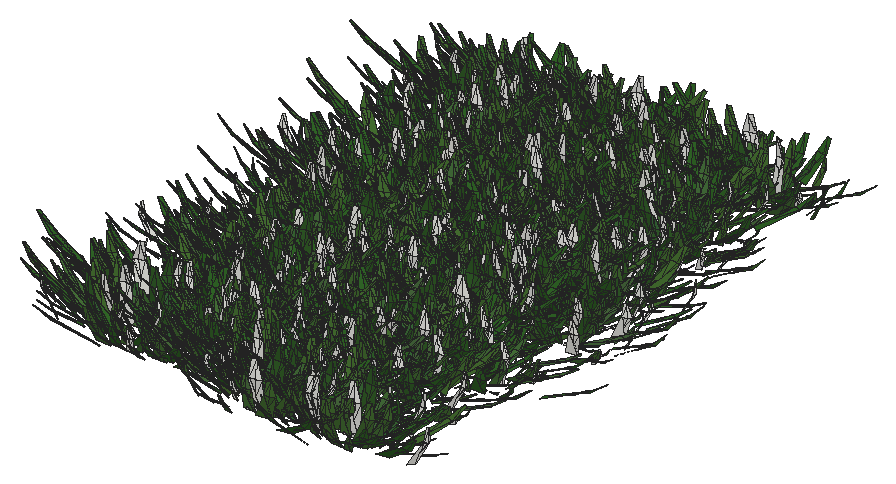
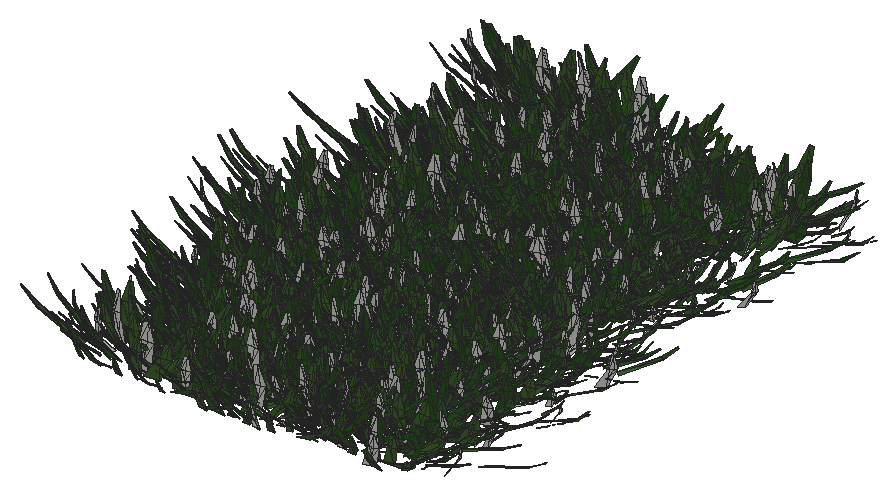
# SketchUp Ruby script. Lengths in inches.
U = 1.inch
M = Sketchup.active_model
def pt(a) = Geom::Point3d.new(a.map { |v| v * U })
def face(e, loops, mat)
  f = e.add_face(loops[0].map { |a| pt(a) })
  loops[1..].each { |l| e.add_face(l.map { |a| pt(a) }).erase! }
  f.material = f.back_material = mat if mat
  f
end
# faces: each face lists its corners as indices into pts; further lists are holes
def faces(e, pts, list, mat = nil) = list.each { |f| face(e, (f[0].is_a?(Array) ? f : [f]).map { |l| l.map { |i| pts[i] } }, mat) }
# xy, xz, yz: faces in a plane at the given z, y or x. An outline is a flat list of corners, or four numbers for a rectangle; further outlines are holes
def ring(l) = l.size == 4 ? [[l[0], l[1]], [l[2], l[1]], [l[2], l[3]], [l[0], l[3]]] : l.each_slice(2).to_a
def flat(e, list, mat, &to3) = list.each { |f| face(e, (f[0].is_a?(Array) ? f : [f]).map { |l| ring(l).map { |u, v| to3.(u, v) } }, mat) }
def xy(e, z, list, mat = nil) = flat(e, list, mat) { |x, y| [x, y, z] }
def xz(e, y, list, mat = nil) = flat(e, list, mat) { |x, z| [x, y, z] }
def yz(e, x, list, mat = nil) = flat(e, list, mat) { |y, z| [x, y, z] }
def lines(e, pts, list) = list.each { |a, b| e.add_line(pt(pts[a]), pt(pts[b])) }
# prism: a flat outline (further loops are holes) pulled along v
def prism(e, loops, v, mat = nil)
  f = face(e, loops, mat); d = Geom::Vector3d.new(v.map { |x| x * U })
  f.pushpull(f.normal.samedirection?(d) ? d.length : -d.length)
end
def box(e, o, s, mat = nil) = prism(e, [[o, [o[0] + s[0], o[1], o[2]], [o[0] + s[0], o[1] + s[1], o[2]], [o[0], o[1] + s[1], o[2]]]], [0, 0, s[2]], mat)
def at(x, y, z, deg = 0) = Geom::Transformation.translation(pt([x, y, z])) * Geom::Transformation.rotation(ORIGIN, Z_AXIS, deg.degrees)
def axes(o, x, y, z) = Geom::Transformation.new([*x, 0, *y, 0, *z, 0, *pt(o).to_a, 1])
def part(name) = M.definitions.add(name)
# library, detail: a bought-in or finely detailed component or shape, given as its bounding box
def library(name, o, s) = part(name).tap { |d| box(d.entities, o, s) }
def detail(e, o, s) = box(e.add_group.entities, o, s)
def put(e, d, t, mat = nil) = e.add_instance(d, t).tap { |i| i.material = mat if mat }
def group(e, t, mat = nil) = e.add_group.tap { |g| g.transformation = t; g.material = mat if mat }.entities
root = M.entities
M.materials.add("Material82").color = [68, 110, 58]
M.materials.add("Material83").color = [48, 90, 38]
M.materials.add("Material84").color = [68, 110, 48]
M.materials.add("Material85").color = [48, 90, 48]
M.materials.add("Material86").color = [58, 110, 58]
M.materials.add("Material87").color = [58, 90, 38]
M.materials.add("Material88").color = [68, 100, 58]
M.materials.add("Material89").color = [48, 100, 38]
c1 = part("grass00")
p = [[-0.6875,0.15,0],[-0.56,0.08,5.52],[-0.04,0.03,2.76],[0.48,-0.02,0],[0.35,-0.02,5.52],[-0.1,-0.14,5.52],
  [-0.12,0.65,8.37],[-0.42,0.65,8.37]]
faces(c1.entities,p,[[0,1,2,3],[3,2,4],[1,5,2],[5,4,2],[1,6,5],[4,5,6],[7,6,1]])
c2 = part("Group16\#1")
put(c2.entities,c1,axes([1.44,-0.61,-0.01],[0.05352,0.12609,0],[-0.10704,0.04543,0.07239],[0.06664,-0.02828,0.11628]),"Material85")
put(c2.entities,c1,axes([0.76,-0.15,-0.01],[0.04676,0.24062,0],[-0.23162,0.04501,0.06642],[0.0652,-0.01267,0.23595]),"Material82")
put(c2.entities,c1,axes([0.79,0.01,-0.01],[-0.00606,0.34651,0],[-0.34381,-0.00602,0.0432],[0.04319,0.00076,0.34386]))
put(c2.entities,c1,axes([1,0.23,-0.01],[-0.07192,0.31144,0],[-0.28722,-0.06632,0.1236],[0.12043,0.02781,0.29478]),"Material84")
put(c2.entities,c1,axes([1.66,0.77,-0.01],[-0.13828,0.29651,0],[-0.21551,-0.1005,0.22471],[0.20365,0.09498,0.23779]),"Material89")
put(c2.entities,c1,axes([0.6875,0.52,-0.01],[-0.18126,0.24051,0],[-0.22746,-0.17142,0.09788],[0.07817,0.05891,0.28481]),"Material84")
put(c2.entities,c1,axes([0.68,0.78,-0.01],[-0.215,0.18688,0],[-0.12385,-0.14248,0.21334],[0.13995,0.16101,0.18878]),"Material82")
put(c2.entities,c1,axes([0.56,1,-0.01],[-0.13756,0.07624,0],[-0.06159,-0.11112,0.0927],[0.04494,0.08108,0.12705]),"Material84")
put(c2.entities,c1,axes([0.2,0.64,-0.01],[-0.23729,0.07254,0],[-0.05711,-0.18681,0.153],[0.04473,0.14632,0.19535]),"Material89")
put(c2.entities,c1,axes([0.0625,0.72,-0.01],[-0.28874,0.02525,0],[-0.02179,-0.24916,0.14647],[0.01276,0.14591,0.25012]),"Material82")
put(c2.entities,c1,axes([-0.08,0.62,-0.01],[-0.34089,-0.04187,0],[0.03255,-0.26504,0.216],[-0.02633,0.21439,0.26703]),"Material89")
put(c2.entities,c1,axes([-0.34,0.98,-0.01],[-0.14314,-0.0493,0],[0.04397,-0.12769,0.06843],[-0.02228,0.0647,0.13505]),"Material89")
put(c2.entities,c1,axes([-0.87,1.45,-0.01],[-0.23488,-0.14114,0],[0.13761,-0.22901,0.06087],[-0.03135,0.05217,0.26717]))
put(c2.entities,c1,axes([-0.72,0.77,-0.01],[-0.14208,-0.13251,0],[0.07209,-0.0773,0.16301],[-0.11118,0.11922,0.1057]),"Material89")
put(c2.entities,c1,axes([-0.62,0.43,-0.01],[-0.14845,-0.21203,0],[0.18654,-0.13061,0.12304],[-0.10079,0.07057,0.22772]),"Material82")
put(c2.entities,c1,axes([-0.68,0.29,-0.01],[-0.13639,-0.32136,0],[0.31723,-0.13464,0.05579],[-0.05136,0.0218,0.34462]),"Material83")
put(c2.entities,c1,axes([-0.64,0.125,-0.01],[-0.0458,-0.23569,0],[0.22124,-0.043,0.08276],[-0.08124,0.01579,0.22538]),"Material86")
put(c2.entities,c1,axes([-1.6,-0.03,-0.01],[0.00576,-0.32897,0],[0.27526,0.00482,0.18018],[-0.18015,-0.00315,0.2753]),"Material84")
put(c2.entities,c1,axes([-1.36,-0.31,-0.01],[0.05718,-0.24765,0],[0.18172,0.04196,0.17267],[-0.16825,-0.03885,0.1865]),"Material89")
put(c2.entities,c1,axes([-1.54,-0.72,-0.01],[0.06537,-0.14017,0],[0.13555,0.06321,0.03939],[-0.0357,-0.01665,0.14956]))
put(c2.entities,c1,axes([-1.19,-0.9,-0.01],[0.09597,-0.12735,0],[0.11214,0.08451,0.07557],[-0.06035,-0.04548,0.14042]),"Material88")
put(c2.entities,c1,axes([-0.47,-0.54,-0.01],[0.11588,-0.10072,0],[0.0618,0.0711,0.12124],[-0.07953,-0.0915,0.0942]))
put(c2.entities,c1,axes([-0.47,-0.84,-0.01],[0.11927,-0.0661,0],[0.06603,0.11913,0.00646],[-0.00313,-0.00565,0.13621]),"Material84")
put(c2.entities,c1,axes([-0.38,-1.24,-0.01],[0.28037,-0.08571,0],[0.0618,0.20215,0.20315],[-0.05939,-0.19428,0.21139]),"Material88")
put(c2.entities,c1,axes([-0.06,-0.66,-0.01],[0.22719,-0.01987,0],[0.01247,0.14255,0.17758],[-0.01547,-0.17691,0.1431]),"Material87")
put(c2.entities,c1,axes([0.11,-0.89,-0.01],[0.14882,0.01828,0],[-0.01058,0.08611,0.12229],[0.01491,-0.12138,0.08676]),"Material85")
put(c2.entities,c1,axes([0.25,-0.72,-0.01],[0.20481,0.07053,0],[-0.06206,0.18022,0.10291],[0.03351,-0.0973,0.1906]),"Material85")
put(c2.entities,c1,axes([0.85,-1.42,-0.01],[0.16481,0.09904,0],[-0.09472,0.15762,0.05616],[0.02893,-0.04814,0.18389]),"Material84")
put(c2.entities,c1,axes([1.01,-1.09,-0.01],[0.21858,0.20385,0],[-0.17495,0.1876,0.15339],[0.10462,-0.11218,0.25652]),"Material89")
put(c2.entities,c1,axes([1.01,-0.71,-0.01],[0.08733,0.12473,0],[-0.06445,0.04512,0.13037],[0.1068,-0.07477,0.07867]),"Material85")
c3 = part("Group15\#1")
put(c3.entities,c2,at(0,0,0))
c4 = part("3darcstudiotree_grass00\#1")
put(c4.entities,c3,at(0,0,0))
put(root,c4,axes([1704.59,960.15,-29.74],[-3.29694,-0.59268,0],[1.38855,-1.20133,-0.0331],[0.08455,-0.07315,1.54531]))
put(root,c4,axes([1703.45,956.93,-29.74],[2.67683,1.25305,0],[-2.64635,0.87925,-0.04423],[-0.18001,0.05981,1.38013]))
put(root,c4,axes([1704.59,979.83,-29.74],[1.85229,-1.14191,0],[3.43107,0.86561,-0.02581],[0.11483,0.02897,1.61243]))
put(root,c4,axes([1705.09,970.66,-29.74],[-0.72323,-1.62263,0],[3.80365,-0.26368,-0.04893],[0.28769,-0.01994,1.72817]))
put(root,c4,axes([1704.83,992.4,-29.74],[-3.72731,0.81099,0],[-1.84954,-1.32207,-0.01481],[-0.0358,-0.02559,1.43556]))
put(root,c4,axes([1704.18,984.05,-29.74],[4.17155,-0.17702,0],[0.50263,1.84221,-0.03237],[0.01504,0.05512,1.52951]))
put(root,c4,axes([1705.72,951.16,-29.74],[-4.25916,-0.67423,0],[1.26133,-1.23925,-0.04034],[0.09396,-0.09232,1.58691]))
put(root,c4,axes([1705.65,976.97,-29.74],[-0.75362,-1.53541,0],[3.24661,-0.24784,-0.00678],[0.04146,-0.00316,1.54322]))
put(root,c4,axes([1706.12,973.3,-29.74],[-2.20792,-1.57829,0],[3.78019,-0.82247,-0.0117],[0.05427,-0.01181,1.7149]))
put(root,c4,axes([1704.51,996.11,-29.74],[1.20267,1.27774,0],[-3.21983,0.47135,-0.04291],[-0.22552,0.03301,1.44315]))
put(root,c4,axes([1705.28,988.91,-29.74],[2.6006,-1.2072,0],[3.21281,1.07644,-0.02612],[0.11842,0.03968,1.8801]))
put(root,c4,axes([1704.72,942.99,-29.74],[-0.33098,1.70392,0],[-3.92143,-0.11847,-0.03234],[-0.20787,-0.00628,1.90052]))
put(root,c4,axes([1704.4,974.61,-29.74],[3.87339,1.05779,0],[-2.14052,1.21905,-0.05103],[-0.17397,0.09908,1.6877]))
put(root,c4,axes([1704.8,943.82,-29.74],[4.23456,-0.44217,0],[1.03247,1.53783,-0.03329],[0.03822,0.05692,1.35616]))
put(root,c4,axes([1705.6875,947.27,-29.74],[-3.02099,1.21639,0],[-3.37871,-1.30508,-0.0181],[-0.07062,-0.02728,1.93624]))
put(root,c4,axes([1706.39,962.33,-29.74],[1.13928,-1.32787,0],[4.00016,0.53378,-0.02846],[0.11467,0.0153,1.34635]))
put(root,c4,axes([1706.87,964.12,-29.74],[1.43898,-1.34623,0],[3.17438,0.52772,-0.03331],[0.18037,0.02999,1.51731]))
put(root,c4,axes([1706.88,985.71,-29.74],[-2.26233,1.10327,0],[-2.6855,-0.85647,-0.00747],[-0.03039,-0.00969,1.35493]))
put(root,c4,axes([1707.01,990.84,-29.74],[0.61227,1.37165,0],[-4.42146,0.30696,-0.06022],[-0.31422,0.02181,1.78296]))
put(root,c4,axes([1707.02,965.45,-29.74],[1.96702,1.06284,0],[-3.17968,0.91525,-0.05552],[-0.21201,0.06102,1.39481]))
put(root,c4,axes([1708.97,995.01,-29.74],[-1.36397,-1.5291,0],[3.40561,-0.47247,-0.03242],[0.15123,-0.02098,1.33794]))
put(root,c4,axes([1710.16,941.96,-29.74],[-3.87962,-0.67736,0],[1.4284,-1.27243,-0.0129],[0.02606,-0.02321,1.31952]))
put(root,c4,axes([1709.1875,980.75,-29.74],[-2.78639,1.08314,0],[-3.04744,-1.21928,-0.00446],[-0.01393,-0.00557,1.44777]))
put(root,c4,axes([1710.14,967.76,-29.74],[-4.49573,0.21611,0],[-0.44378,-1.43584,-0.03065],[-0.02667,-0.0863,1.97713]))
put(root,c4,axes([1710.64,991.92,-29.74],[-1.74555,-1.44076,0],[3.95857,-0.74592,-0.00689],[0.03295,-0.00621,1.74288]))
put(root,c4,axes([1710.59,987.44,-29.74],[-3.15245,-0.45856,0],[1.56973,-1.67838,-0.02933],[0.05139,-0.05494,1.72129]))
put(root,c4,axes([1709.32,996.1875,-29.74],[4.34464,0.20061,0],[-0.52956,1.78372,-0.02723],[-0.01491,0.05022,1.60719]))
put(root,c4,axes([1709.7,946.51,-29.74],[3.87508,-0.19158,0],[0.55593,1.74888,-0.03701],[0.02742,0.08626,1.99511]))
put(root,c4,axes([1709.46,973.63,-29.74],[4.00255,0.79486,0],[-1.95042,1.52752,-0.03278],[-0.08544,0.06692,1.8841]))
put(root,c4,axes([1710.78,966.61,-29.74],[1.64847,-1.35078,0],[4.23243,0.80334,-0.06017],[0.26789,0.05085,1.73941]))
put(root,c4,axes([1710.63,957.09,-29.74],[2.33049,-1.15129,0],[2.65609,0.83622,-0.01018],[0.04728,0.01488,1.51436]))
put(root,c4,axes([1709.875,983.62,-29.74],[3.64852,0.24315,0],[-0.61045,1.42466,-0.04218],[-0.04748,0.11082,1.85529]))
put(root,c4,axes([1711.36,952.86,-29.74],[-1.10259,-1.32087,0],[4.19794,-0.54501,-0.05688],[0.29749,-0.03862,1.82396]))
put(root,c4,axes([1709.81,962.37,-29.74],[4.20126,0.39077,0],[-0.91213,1.52518,-0.02883],[-0.04091,0.06841,1.84132]))
put(root,c4,axes([1710.81,951.28,-29.74],[2.88399,-0.92183,0],[2.75264,1.33938,-0.02341],[0.07157,0.03482,1.59067]))
put(root,c4,axes([1711.875,974.9,-29.74],[-3.28835,-0.7389,0],[1.7462,-1.20864,-0.01205],[0.03007,-0.02081,1.33255]))
put(root,c4,axes([1711.99,955.34,-29.74],[-3.05685,-0.82947,0],[2.14696,-1.23058,-0.02104],[0.07287,-0.04177,1.73448]))
put(root,c4,axes([1712,985.56,-29.74],[-2.64127,-0.90818,0],[2.55598,-1.15614,-0.03875],[0.14904,-0.06742,1.70607]))
put(root,c4,axes([1711.27,959.7,-29.74],[2.49775,-0.87161,0],[2.87959,1.28342,-0.04815],[0.19249,0.08579,1.9649]))
put(root,c4,axes([1711.02,989.8,-29.74],[3.57061,0.64267,0],[-1.40632,1.21522,-0.03533],[-0.10777,0.09312,1.86502]))
put(root,c4,axes([1711.87,970.9375,-29.74],[3.75674,0.29184,0],[-0.86575,1.73332,-0.03192],[-0.02673,0.05352,1.45488]))
put(root,c4,axes([1712.22,978.89,-29.74],[-0.44896,1.44211,0],[-4.03082,-0.19517,-0.03564],[-0.19872,-0.00962,1.71014]))
put(root,c4,axes([1711.87,948.04,-29.74],[4.11072,0.52115,0],[-1.12592,1.38127,-0.00634],[-0.01225,0.01503,1.74238]))
put(root,c4,axes([1712.75,963.79,-29.74],[3.24027,-0.98547,0],[2.31887,1.18584,-0.00737],[0.02262,0.01157,1.42978]))
put(root,c4,axes([1712.1,943.9,-29.74],[0.47172,1.49628,0],[-3.52699,0.17294,-0.00588],[-0.02991,0.00147,1.36568]))
put(root,c4,axes([1712.01,977.6,-29.74],[2.55644,1.08061,0],[-3.46336,1.27432,-0.03325],[-0.10953,0.0403,1.59934]))
put(root,c4,axes([1714.31,994.85,-29.74],[-3.55761,-0.37183,0],[0.9234,-1.37408,-0.01321],[0.02436,-0.03625,1.9444]))
put(root,c4,axes([1714.61,962.64,-29.74],[-1.58706,-1.22315,0],[3.88697,-0.78439,-0.02541],[0.09132,-0.01843,1.32108]))
put(root,c4,axes([1714.41,979.85,-29.74],[0.37581,-1.33084,0],[4.05324,0.17801,-0.00391],[0.01773,0.00078,1.39627]))
put(root,c4,axes([1714.2,973.54,-29.74],[0.29138,-1.80133,0],[3.99838,0.10059,-0.05413],[0.25015,0.00629,1.39055]))
put(root,c4,axes([1714.4,959.01,-29.74],[0.60335,-1.83981,0],[4.64218,0.23677,-0.05291],[0.19949,0.01017,1.33374]))
put(root,c4,axes([1714.64,951.6,-29.74],[-4.16919,-0.21002,0],[0.49933,-1.5417,-0.0157],[0.01299,-0.04011,1.92971]))
put(root,c4,axes([1714.71,992.99,-29.74],[0.3233,-1.61244,0],[3.70268,0.11546,-0.00365],[0.02017,0.00063,1.54435]))
put(root,c4,axes([1714.77,970.72,-29.74],[2.70248,-1.34249,0],[3.67105,1.14936,-0.06314],[0.18316,0.05735,1.30132]))
put(root,c4,axes([1714.93,949.09,-29.74],[-3.51608,0.58555,0],[-1.76508,-1.64843,-0.01449],[-0.02729,-0.02549,1.64714]))
put(root,c4,axes([1716.21,996.89,-29.74],[-1.97159,-1.316,0],[4.00038,-0.93213,-0.05519],[0.24758,-0.05769,1.81465]))
put(root,c4,axes([1714.34,964.21,-29.74],[2.05839,1.31648,0],[-3.03228,0.73739,-0.00763],[-0.03853,0.00937,1.58363]))
put(root,c4,axes([1714.75,976.98,-29.74],[3.97377,-0.0043,0],[0.0116,1.66593,-0.02008],[0.00028,0.04042,1.61638]))
put(root,c4,axes([1714.875,953.96,-29.74],[0.70204,1.43301,0],[-3.58325,0.27302,-0.03785],[-0.19362,0.01475,1.42505]))
put(root,c4,axes([1716.53,989.69,-29.74],[-3.33443,-0.23634,0],[0.70723,-1.55188,-0.01818],[0.01451,-0.03184,1.35222]))
put(root,c4,axes([1716.86,957.45,-29.74],[-4.02551,-0.90949,0],[2.09135,-1.43967,-0.04075],[0.0999,-0.06877,1.55523]))
put(root,c4,axes([1715.01,975.52,-29.74],[4.20535,0.69684,0],[-1.48182,1.39084,-0.00848],[-0.02193,0.02058,1.91304]))
put(root,c4,axes([1715.22,955.63,-29.74],[3.86131,0.54377,0],[-1.4335,1.58316,-0.00059],[-0.00108,0.0012,1.74794]))
put(root,c4,axes([1716.58,983.61,-29.74],[2.33801,-1.27151,0],[3.45385,0.98774,-0.00976],[0.0468,0.01338,1.89325]))
put(root,c4,axes([1716.91,985.51,-29.74],[-0.84806,-1.31842,0],[3.86352,-0.38651,-0.05601],[0.32758,-0.03277,1.80254]))
put(root,c4,axes([1716.92,969.14,-29.74],[2.53276,-1.11904,0],[3.44801,1.21375,-0.02458],[0.09462,0.03331,1.78746]))
put(root,c4,axes([1717.91,981.83,-29.74],[-3.79387,-0.48377,0],[1.38418,-1.6883,-0.04655],[0.0671,-0.08184,1.58019]))
put(root,c4,axes([1716.64,946.28,-29.74],[3.58882,-0.43849,0],[1.01017,1.28588,-0.04073],[0.06773,0.08621,1.43775]))
put(root,c4,axes([1716.68,944.61,-29.74],[1.5336,1.30723,0],[-4.13356,0.75421,-0.03574],[-0.18177,0.03317,1.91331]))
put(root,c4,axes([1717.13,988.3125,-29.74],[4.25696,0.81021,0],[-1.71809,1.40397,-0.05424],[-0.1086,0.08874,1.36476]))
put(root,c4,axes([1718.27,965.67,-29.74],[1.26993,-1.49927,0],[3.12751,0.41201,-0.03453],[0.23339,0.03075,1.76116]))
put(root,c4,axes([1718.33,942.89,-29.74],[0.88446,1.28365,0],[-3.4154,0.366,-0.02204],[-0.14997,0.01607,1.87051]))
put(root,c4,axes([1719.91,957.21,-29.74],[-4.2844,-0.03587,0],[0.08793,-1.63328,-0.04949],[0.00646,-0.12004,1.9102]))
put(root,c4,axes([1720.89,986.64,-29.74],[-1.79663,-1.22383,0],[3.52148,-0.80403,-0.02105],[0.11606,-0.0265,1.94345]))
put(root,c4,axes([1720.08,983.79,-29.74],[-3.1837,0.9292,0],[-2.49148,-1.32767,-0.01624],[-0.05606,-0.02987,1.82169]))
put(root,c4,axes([1720.52,963.31,-29.74],[2.23016,-1.08828,0],[2.80047,0.89256,-0.01488],[0.0583,0.01858,1.35946]))
put(root,c4,axes([1721.32,981.42,-29.74],[-2.22834,-1.37792,0],[3.47538,-0.87412,-0.04256],[0.18098,-0.04552,1.55835]))
put(root,c4,axes([1720.1,992.89,-29.74],[3.33835,-0.04276,0],[0.15045,1.82678,-0.05593],[0.00839,0.10182,1.60461]))
put(root,c4,axes([1721.44,989.77,-29.74],[0.7854,-1.46662,0],[3.6757,0.30614,-0.00249],[0.01359,0.00113,1.57305]))
put(root,c4,axes([1720.77,996.89,-29.74],[-3.47223,1.22215,0],[-3.01377,-1.3317,-0.01139],[-0.0395,-0.01745,1.76647]))
put(root,c4,axes([1721.92,995.18,-29.74],[-0.62966,-1.28695,0],[4.54348,-0.34574,-0.02161],[0.1197,-0.00911,1.95654]))
put(root,c4,axes([1721.68,952.93,-29.74],[1.31559,-1.26739,0],[3.71813,0.60026,-0.00546],[0.02236,0.00361,1.33158]))
put(root,c4,axes([1720.42,977.52,-29.74],[0.91997,1.29984,0],[-3.25818,0.35865,-0.02635],[-0.1448,0.01594,1.4463]))
put(root,c4,axes([1720.86,987.94,-29.74],[-2.04292,1.4828,0],[-3.7482,-0.80316,-0.0267],[-0.09668,-0.02072,1.31753]))
put(root,c4,axes([1722,940.42,-29.74],[1.12764,-1.73077,0],[4.18377,0.42395,-0.01129],[0.06303,0.00639,1.86628]))
put(root,c4,axes([1720.45,975.1875,-29.74],[3.72756,0.95688,0],[-1.9535,1.18357,-0.02904],[-0.10466,0.06341,1.7729]))
put(root,c4,axes([1721.18,972.29,-29.74],[3.3945,-0.58791,0],[1.6844,1.5126,-0.00525],[0.01109,0.00996,1.64886]))
put(root,c4,axes([1721.34,978.79,-29.74],[3.30024,-0.68967,0],[2.06464,1.53659,-0.00115],[0.00232,0.00173,1.42878]))
put(root,c4,axes([1720.82,960.32,-29.74],[3.05854,0.58726,0],[-2.04234,1.65433,-0.05845],[-0.11264,0.09124,1.53958]))
put(root,c4,axes([1722.5,950.68,-29.74],[-4.47684,0.54828,0],[-1.1065,-1.40519,-0.03919],[-0.07055,-0.08959,1.69748]))
put(root,c4,axes([1721.36,968.63,-29.74],[4.02075,-0.11832,0],[0.27482,1.45248,-0.02534],[0.01078,0.05696,1.58232]))
put(root,c4,axes([1721.92,945.09,-29.74],[3.57543,-0.38769,0],[0.94849,1.36047,-0.03828],[0.05948,0.08532,1.57185]))
put(root,c4,axes([1721.75,971.41,-29.74],[3.70563,0.39578,0],[-0.96164,1.40032,-0.0432],[-0.06214,0.09049,1.51727]))
put(root,c4,axes([1722.5,947.01,-29.74],[-2.1552,1.3099,0],[-3.57978,-0.91604,-0.05659],[-0.20761,-0.05313,1.39892]))
put(root,c4,axes([1723.58,966.39,-29.74],[2.80865,-0.79423,0],[2.35611,1.29587,-0.04704],[0.15431,0.08487,1.70604]))
put(root,c4,axes([1722.77,942.25,-29.74],[3.02481,0.98705,0],[-2.84435,1.35567,-0.00662],[-0.02068,0.00986,1.63949]))
put(root,c4,axes([1723.59,961.53,-29.74],[4.31211,0.22009,0],[-0.60247,1.83583,-0.04718],[-0.02535,0.07723,1.4726]))
put(root,c4,axes([1723.85,948.86,-29.74],[0.84595,1.74988,0],[-3.45616,0.25986,-0.03349],[-0.2005,0.01508,1.60736]))
put(root,c4,axes([1725.34,949.62,-29.74],[-2.74028,-0.81988,0],[2.08475,-1.08371,-0.01586],[0.05642,-0.02933,1.52204]))
put(root,c4,axes([1723.82,955.56,-29.74],[3.77018,0.78532,0],[-1.755,1.3104,-0.05015],[-0.15166,0.11324,1.82381]))
put(root,c4,axes([1725.36,969.24,-29.74],[3.19182,-1.13301,0],[2.43556,1.06713,-0.02235],[0.10598,0.04644,1.93391]))
put(root,c4,axes([1725.98,975.73,-29.74],[2.31636,-1.46039,0],[3.68995,0.91026,-0.01393],[0.05236,0.01292,1.44657]))
put(root,c4,axes([1726.03,995.14,-29.74],[-3.95397,0.70682,0],[-1.69994,-1.479,-0.00714],[-0.01245,-0.01084,1.30481]))
put(root,c4,axes([1726.3125,962.23,-29.74],[1.88589,-1.60822,0],[4.27567,0.77981,-0.01],[0.0511,0.00932,1.98774]))
put(root,c4,axes([1725.53,960.27,-29.74],[-1.85089,1.19146,0],[-2.90652,-0.70224,-0.01687],[-0.07661,-0.01851,1.36079]))
put(root,c4,axes([1726.77,941.74,-29.74],[1.40551,-1.64885,0],[4.26228,0.56508,-0.02131],[0.10181,0.0135,1.69918]))
put(root,c4,axes([1726.13,955.81,-29.74],[2.41246,-1.41032,0],[3.04441,0.80995,-0.04469],[0.24595,0.06543,1.8275]))
put(root,c4,axes([1726.05,997.6,-29.74],[-0.9909,1.30306,0],[-3.23471,-0.38257,-0.04553],[-0.22482,-0.02659,1.30482]))
put(root,c4,axes([1727.24,973.16,-29.74],[-2.9141,-1.11595,0],[2.66035,-1.08046,-0.03796],[0.14613,-0.05935,1.58175]))
put(root,c4,axes([1725.67,987.78,-29.74],[-0.05283,1.30539,0],[-4.56112,-0.02871,-0.04794],[-0.23084,-0.00145,1.64652]))
put(root,c4,axes([1726.76,976.38,-29.74],[1.60686,-1.51832,0],[3.56667,0.58707,-0.05171],[0.27066,0.04455,1.64301]))
put(root,c4,axes([1727.9,990.74,-29.74],[-1.63027,-1.73131,0],[4.11958,-0.60332,-0.00006],[0.00033,-0.00005,1.81412]))
put(root,c4,axes([1726.27,992.01,-29.74],[0.46872,1.37145,0],[-4.27579,0.22728,-0.05207],[-0.28533,0.01517,1.7882]))
put(root,c4,axes([1727.88,950.47,-29.74],[-3.00354,-1.31894,0],[3.37135,-1.19405,-0.05274],[0.22952,-0.08129,1.98669]))
put(root,c4,axes([1726.23,944.83,-29.74],[0.98392,1.60393,0],[-4.31274,0.41147,-0.01063],[-0.04621,0.00441,1.48723]))
put(root,c4,axes([1727.01,985.38,-29.74],[4.05845,0.38101,0],[-1.01694,1.68476,-0.06215],[-0.0714,0.11828,1.63292]))
put(root,c4,axes([1728.83,979.07,-29.74],[-3.29654,-0.72222,0],[2.17338,-1.54289,-0.02959],[0.0707,-0.05019,1.65043]))
put(root,c4,axes([1727.24,983.92,-29.74],[1.47468,1.38827,0],[-3.83437,0.63347,-0.03717],[-0.17802,0.02941,1.61797]))
put(root,c4,axes([1727.25,964.12,-29.74],[2.9165,0.98147,0],[-2.52132,1.16527,-0.03219],[-0.13562,0.06268,1.88986]))
put(root,c4,axes([1727.04,945.96,-29.74],[2.31946,1.24356,0],[-3.54601,1.02866,-0.02079],[-0.06877,0.01995,1.35493]))
put(root,c4,axes([1729.25,981.77,-29.74],[-4.41332,-0.66754,0],[1.63018,-1.67623,-0.02874],[0.04038,-0.04152,1.33872]))
put(root,c4,axes([1728.72,971.08,-29.74],[-2.71187,1.03836,0],[-2.98144,-1.21104,-0.01854],[-0.0717,-0.02913,1.78092]))
put(root,c4,axes([1728.69,957.99,-29.74],[4.10034,-0.52862,0],[1.2552,1.51427,-0.04269],[0.08479,0.10229,1.93529]))
put(root,c4,axes([1729.3,953.07,-29.74],[2.75881,-1.06303,0],[3.05708,1.23394,-0.03867],[0.14354,0.05794,1.7417]))
put(root,c4,axes([1728.93,966.5625,-29.74],[-0.60337,1.5081,0],[-3.83662,-0.23874,-0.0149],[-0.0971,-0.00604,1.9212]))
put(root,c4,axes([1731.28,972.65,-29.74],[-3.93883,-1.01936,0],[1.86002,-1.11781,-0.04657],[0.18505,-0.11121,1.84036]))
put(root,c4,axes([1730.99,942.04,-29.74],[1.31732,-1.5277,0],[3.94533,0.52911,-0.01889],[0.1126,0.0151,1.96679]))
put(root,c4,axes([1730.89,979.33,-29.74],[2.55399,-1.11237,0],[2.83561,1.01258,-0.04299],[0.17745,0.06336,1.59659]))
put(root,c4,axes([1731.79,940.71,-29.74],[-3.03372,-1.40875,0],[3.08967,-1.03482,-0.05304],[0.26,-0.08708,1.95407]))
put(root,c4,axes([1731.74,981.73,-29.74],[-4.27576,-0.00967,0],[0.01971,-1.35519,-0.00073],[0.00002,-0.00168,1.50826]))
put(root,c4,axes([1731.09,983.67,-29.74],[-2.10798,1.40451,0],[-3.51427,-0.82033,-0.03668],[-0.20421,-0.04767,1.98009]))
put(root,c4,axes([1731.49,958.95,-29.74],[-3.10894,1.29688,0],[-2.64938,-0.9878,-0.02847],[-0.10631,-0.03964,1.40417]))
put(root,c4,axes([1731.93,985.5,-29.74],[-3.43779,0.5694,0],[-1.45981,-1.37078,-0.01995],[-0.04437,-0.04166,1.62326]))
put(root,c4,axes([1731.33,997.06,-29.74],[-1.73682,1.47733,0],[-4.1333,-0.75577,-0.04346],[-0.21523,-0.03935,1.86413]))
put(root,c4,axes([1731.59,949.3125,-29.74],[-2.48253,1.23787,0],[-2.67891,-0.83558,-0.01059],[-0.04346,-0.01356,1.33934]))
put(root,c4,axes([1732.55,968.86,-29.74],[-4.54038,0.15264,0],[-0.30495,-1.41082,-0.04632],[-0.02774,-0.12834,1.89764]))
put(root,c4,axes([1730.96,988.71,-29.74],[3.62862,0.35052,0],[-1.11939,1.8023,-0.01455],[-0.01942,0.03128,1.97892]))
put(root,c4,axes([1733.47,969.85,-29.74],[-4.13743,-0.67569,0],[1.3247,-1.26157,-0.00358],[0.00873,-0.00832,1.65637]))
put(root,c4,axes([1732.56,976.7,-29.74],[-1.22945,1.37189,0],[-3.12548,-0.43563,-0.03966],[-0.20868,-0.02909,1.38647]))
put(root,c4,axes([1733.04,964.71,-29.74],[-3.50072,1.23157,0],[-2.52643,-1.11691,-0.04505],[-0.14682,-0.06491,1.39266]))
put(root,c4,axes([1733.98,974.22,-29.74],[-1.35898,-1.3893,0],[3.82798,-0.58237,-0.03571],[0.20852,-0.03172,1.92492]))
put(root,c4,axes([1732.58,994.8,-29.74],[1.95907,1.41788,0],[-3.34699,0.71925,-0.025],[-0.15312,0.03291,1.99255]))
put(root,c4,axes([1734.23,966.24,-29.74],[-4.10859,0.05118,0],[-0.12582,-1.57107,-0.03959],[-0.00691,-0.08629,1.65212]))
put(root,c4,axes([1733.375,955.9,-29.74],[3.60532,-0.46019,0],[1.33734,1.62954,-0.01611],[0.02411,0.02937,1.58139]))
